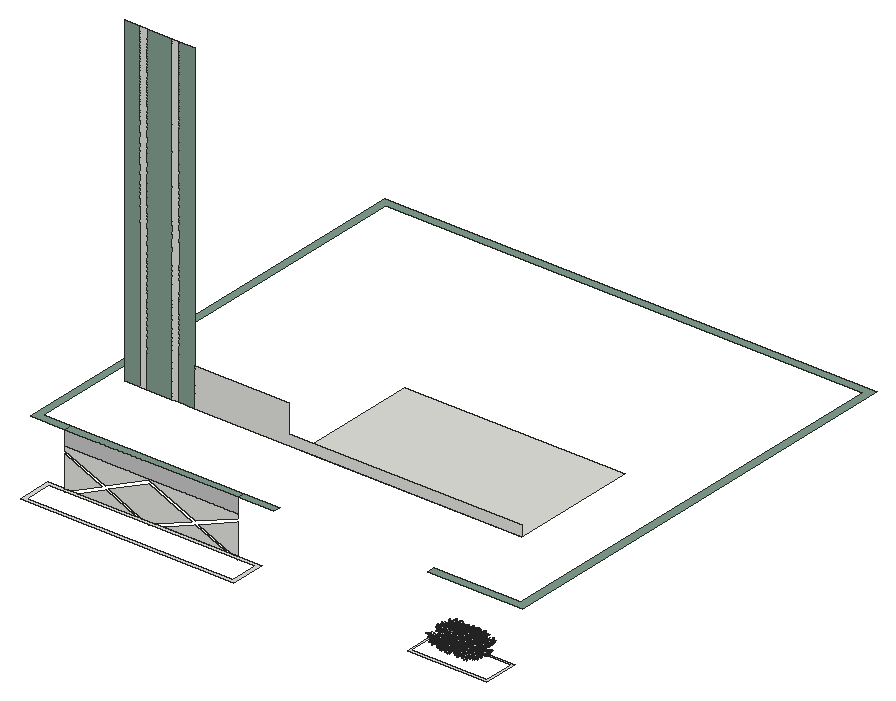
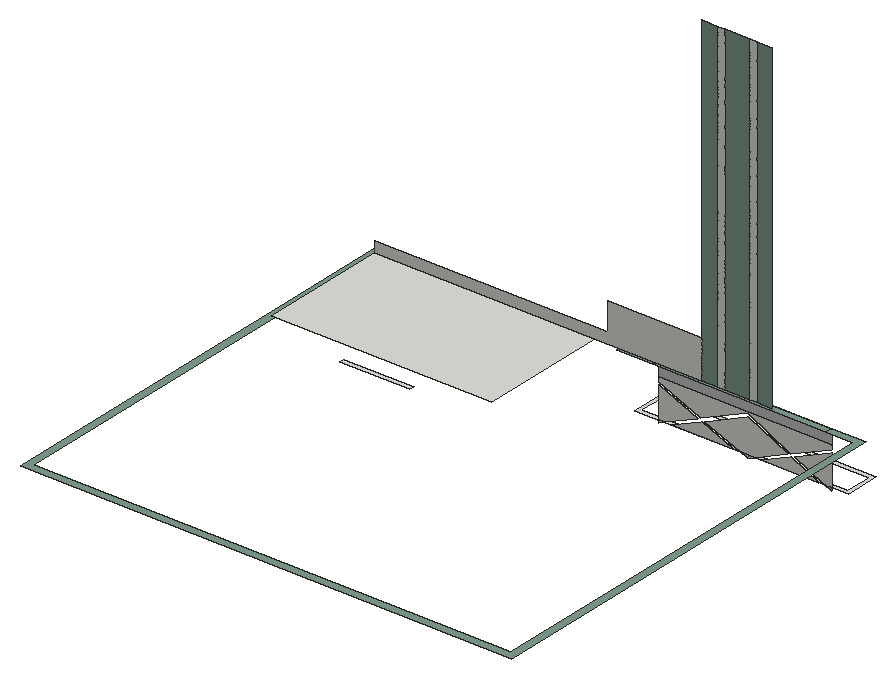
# SketchUp Ruby script. Lengths in inches.
U = 1.inch
M = Sketchup.active_model
def pt(a) = Geom::Point3d.new(a.map { |v| v * U })
def face(e, loops, mat)
  f = e.add_face(loops[0].map { |a| pt(a) })
  loops[1..].each { |l| e.add_face(l.map { |a| pt(a) }).erase! }
  f.material = f.back_material = mat if mat
  f
end
# faces: each face lists its corners as indices into pts; further lists are holes
def faces(e, pts, list, mat = nil) = list.each { |f| face(e, (f[0].is_a?(Array) ? f : [f]).map { |l| l.map { |i| pts[i] } }, mat) }
# xy, xz, yz: faces in a plane at the given z, y or x. An outline is a flat list of corners, or four numbers for a rectangle; further outlines are holes
def ring(l) = l.size == 4 ? [[l[0], l[1]], [l[2], l[1]], [l[2], l[3]], [l[0], l[3]]] : l.each_slice(2).to_a
def flat(e, list, mat, &to3) = list.each { |f| face(e, (f[0].is_a?(Array) ? f : [f]).map { |l| ring(l).map { |u, v| to3.(u, v) } }, mat) }
def xy(e, z, list, mat = nil) = flat(e, list, mat) { |x, y| [x, y, z] }
def xz(e, y, list, mat = nil) = flat(e, list, mat) { |x, z| [x, y, z] }
def yz(e, x, list, mat = nil) = flat(e, list, mat) { |y, z| [x, y, z] }
def lines(e, pts, list) = list.each { |a, b| e.add_line(pt(pts[a]), pt(pts[b])) }
# prism: a flat outline (further loops are holes) pulled along v
def prism(e, loops, v, mat = nil)
  f = face(e, loops, mat); d = Geom::Vector3d.new(v.map { |x| x * U })
  f.pushpull(f.normal.samedirection?(d) ? d.length : -d.length)
end
def box(e, o, s, mat = nil) = prism(e, [[o, [o[0] + s[0], o[1], o[2]], [o[0] + s[0], o[1] + s[1], o[2]], [o[0], o[1] + s[1], o[2]]]], [0, 0, s[2]], mat)
def at(x, y, z, deg = 0) = Geom::Transformation.translation(pt([x, y, z])) * Geom::Transformation.rotation(ORIGIN, Z_AXIS, deg.degrees)
def axes(o, x, y, z) = Geom::Transformation.new([*x, 0, *y, 0, *z, 0, *pt(o).to_a, 1])
def part(name) = M.definitions.add(name)
# library, detail: a bought-in or finely detailed component or shape, given as its bounding box
def library(name, o, s) = part(name).tap { |d| box(d.entities, o, s) }
def detail(e, o, s) = box(e.add_group.entities, o, s)
def put(e, d, t, mat = nil) = e.add_instance(d, t).tap { |i| i.material = mat if mat }
def group(e, t, mat = nil) = e.add_group.tap { |g| g.transformation = t; g.material = mat if mat }.entities
root = M.entities
M.materials.add("[Color H08]").color = [130, 158, 143]
M.materials.add("[Color M02]").color = [198, 198, 198]
c1 = part("Plane.003")
p = [[-13.75,10.1875,13.53],[-8.85,45.75,19.16],[-0.05,76.91,20.56],[0.09,-0.03,-0.02],[7.48,49.37,17.16],[14.16,9.16,9.9]]
faces(c1.entities,p,[[0,1,2,3],[4,5,3,2]])
c2 = part("spirea_leaf")
put(c2.entities,c1,at(0,0,0))
c3 = part("Plane.002")
p = [[-2.92,82.99,124.67],[-2.92,-0.79,0],[2.92,-0.79,0],[2.92,82.99,124.67],[2.92,149.28,292.15],[-2.92,149.28,292.15],
  [2.92,182.43,464.87],[-2.92,182.43,464.87]]
faces(c3.entities,p,[[0,1,2,3],[3,4,5,0],[5,4,6],[5,6,7]])
c4 = part("spirea_stem")
put(c4.entities,c3,at(0,0,0))
c5 = part("spirea_single")
put(c5.entities,c2,axes([61.07,82.24,152.17],[-0.04534,0.68195,-0.35141],[-0.74248,-0.12758,-0.15177],[-0.19302,0.33055,0.66639]))
put(c5.entities,c2,axes([59.72,73.38,127.91],[0.28617,0.56014,-0.10586],[-0.56688,0.26713,-0.11894],[-0.06012,0.14744,0.61766]))
put(c5.entities,c4,axes([60.19,1.84,0],[0.3441,0,0],[0,0.62,0],[0,0,0.62]))
put(c5.entities,c2,axes([59.67,34.88,53.33],[0.45126,0.21625,-0.53161],[-0.52806,0.42133,-0.27684],[0.2248,0.55563,0.41684]))
put(c5.entities,c2,axes([59.72,42.6,61.76],[0.43966,-0.56732,0.27467],[0.6265,0.43009,-0.11449],[-0.0692,0.28942,0.70855]))
put(c5.entities,c2,axes([60.64,103.19,225.26],[-0.35027,-0.4893,-0.00056],[0.48916,-0.35019,0.01365],[-0.01142,0.00749,0.60159]))
put(c5.entities,c2,axes([59.49,100.02,211.41],[0.59184,-0.32302,0],[0.323,0.59181,-0.00668],[0.0032,0.00586,0.67422]))
put(c5.entities,c2,axes([60.71,98.4,200.52],[0.37279,0.59177,-0.19096],[-0.61923,0.37358,-0.05117],[0.05663,0.18942,0.69752]))
put(c5.entities,c2,axes([60.46,79.17,144.19],[-0.69777,0.02304,-0.21354],[-0.09001,-0.69041,0.21963],[-0.195,0.23624,0.6627]))
put(c5.entities,c2,axes([59.53,75.43,133.01],[0.51977,-0.50179,-0.10513],[0.47164,0.52669,-0.18209],[0.201,0.06172,0.69914]))
put(c5.entities,c2,axes([61.85,65.23,103.75],[-0.33765,-0.67856,0.12705],[0.68306,-0.34887,-0.04799],[0.10005,0.09184,0.75641]))
put(c5.entities,c2,axes([59.93,92.9,176.87],[0.03118,-0.56709,0.29033],[0.62588,0.08155,0.09208],[-0.11899,0.28038,0.56044]))
put(c5.entities,c2,axes([60.8125,96.09,190.88],[-0.43546,0.45576,-0.27755],[-0.47188,-0.49616,-0.07437],[-0.24915,0.14314,0.62595]))
put(c5.entities,c2,axes([61.06,86.21,159.17],[0.68151,0.1886,0.10384],[-0.14294,0.65414,-0.24995],[-0.161,0.21757,0.66147]))
put(c5.entities,c2,axes([61.02,103.72,233.5],[0.15025,0.6695,-0.05975],[-0.66771,0.14162,-0.09212],[-0.07726,0.07802,0.67994]))
put(c5.entities,c2,axes([59.84,60.39,94.71],[0.69689,-0.19053,-0.10513],[0.16077,0.68848,-0.18209],[0.14666,0.15067,0.69914]))
put(c5.entities,c2,axes([60.35,111.25,265.8],[-0.44527,0.00464,-0.00041],[-0.00465,-0.44516,0.0101],[-0.00031,0.0101,0.44518]))
put(c5.entities,c2,axes([62.04,106.17,241.79],[0.58725,0,0],[0,0.58493,-0.0522],[0,0.0522,0.58493]))
put(c5.entities,c2,axes([61.05,108.11,252.87],[-0.04027,-0.58443,0.33381],[0.6723,-0.01918,0.04751],[-0.03168,0.33568,0.58389]))
c6 = part("spirea_noflower")
put(c6.entities,c4,axes([7.4375,15.95,0.02],[-0.05138,-0.02266,0],[0.04001,-0.09072,0.02017],[-0.00814,0.01846,0.09915]))
put(c6.entities,c2,axes([10.92,7.8,33.61],[0.09808,-0.04627,-0.02956],[0.03942,0.10146,-0.02804],[0.03822,0.0141,0.10476]))
put(c6.entities,c2,axes([10.66,8.28,28.22],[-0.09096,-0.06939,0.02274],[0.06684,-0.09374,-0.01869],[0.0294,-0.00154,0.11286]))
put(c6.entities,c2,axes([10.82,7.9375,40.67],[0.02156,-0.10964,0.01223],[0.11005,0.02051,-0.01012],[0.00764,0.01391,0.11128]))
put(c6.entities,c2,axes([10.02,10.22,17.07],[-0.11498,-0.02115,-0.02301],[0.02282,-0.11675,-0.00672],[-0.02136,-0.01089,0.11671]))
put(c6.entities,c2,axes([10.95,7.79,39.34],[0.02073,0.09465,-0.01601],[-0.09582,0.01943,-0.00921],[-0.00571,0.01757,0.09645]))
put(c6.entities,c2,axes([9.92,9.65,18.67],[0.00496,0.12531,-0.00176],[-0.12388,0.00463,-0.01903],[-0.01894,0.00249,0.12396]))
put(c6.entities,c2,axes([11.03,7.9,31.26],[-0.04507,0.08957,0.02798],[-0.0894,-0.05041,0.01738],[0.0285,-0.01651,0.09875]))
put(c6.entities,c2,axes([8.95,12.73,9.62],[-0.04645,-0.07719,-0.07798],[0.10968,-0.03512,-0.03057],[-0.00318,-0.0837,0.08474]))
put(c6.entities,c2,axes([10.44,9.32,22.8],[-0.00519,-0.10396,0.0013],[0.10345,-0.00529,-0.01033],[0.01038,0.00077,0.10358]))
put(c6.entities,c2,axes([9.33,11.85,11.22],[-0.10587,0.06223,0.02547],[-0.06429,-0.1076,-0.00432],[0.01971,-0.0167,0.12273]))
put(c6.entities,c2,axes([10.09,9.85,19.95],[0.08489,-0.07402,0.03033],[0.07003,0.09014,0.02399],[-0.03866,0.00075,0.11004]))
put(c6.entities,c2,axes([10.96,7.75,35.23],[-0.01497,-0.11683,-0.01129],[0.11725,-0.0154,0.00397],[-0.00539,-0.01068,0.11771]))
put(c6.entities,c2,axes([11.1,7.92,37.02],[-0.10922,0.00829,-0.01051],[-0.00995,-0.10807,0.01819],[-0.00895,0.019,0.10801]))
put(c6.entities,c2,axes([10.5,8.65,26.97],[0.0554,-0.10726,-0.03401],[0.10463,0.06305,-0.02842],[0.0414,-0.01582,0.11733]))
put(c6.entities,c2,axes([10.49,8.91,25.59],[0.10848,0.03623,-0.0334],[-0.034,0.11349,0.01266],[0.03566,-0.002,0.11367]))
put(c6.entities,c2,axes([10.54,9.18,23.68],[-0.10862,0.03606,-0.03314],[-0.03404,-0.11355,-0.01198],[-0.03521,-0.00146,0.11382]))
put(c6.entities,c2,axes([10.72,7.76,42.08],[-0.08769,-0.03868,0],[0.03843,-0.08714,0.01068],[-0.00431,0.00977,0.09524]))
put(c6.entities,c2,axes([10.85,7.87,43.91],[-0.03609,0.09811,0.03437],[-0.10225,-0.04006,0.00697],[0.01873,-0.02965,0.1043]))
put(c6.entities,c2,axes([10.98,7.84,46.08],[0.06679,0.02863,0.00008],[-0.02817,0.06574,-0.01287],[-0.00515,0.01179,0.07152]))
put(c6.entities,c2,axes([10.8,7.97,48.125],[-0.06893,0.0419,0.00009],[-0.04141,-0.06814,0.0122],[0.00642,0.01038,0.07974]))
put(c6.entities,c2,axes([10.94,7.82,49.1],[0.01894,-0.07016,0.00008],[0.05795,0.01569,0.04095],[-0.03956,-0.0106,0.06003]))
c7 = part("Spirea")
put(c7.entities,c5,axes([20.99,29.53,3.1875],[0.01954,-0.091,-0.02329],[0.08848,0.02778,-0.02423],[0.03497,-0.01946,0.07433]))
put(c7.entities,c5,axes([16.1875,23.97,1.65],[0.09656,0,0],[0,0.09656,0],[0,0,0.08111]))
put(c7.entities,c6,axes([35.43,25.1,-1.16],[-0.42763,0.26514,-0.05489],[-0.21558,-0.25326,0.32187],[0.16762,0.35071,0.27393]))
put(c7.entities,c6,axes([22.85,19.9,0.53],[0.4898,0.21094,-0.05818],[-0.15904,0.4504,0.20754],[0.15492,-0.20455,0.39699]))
put(c7.entities,c6,axes([25.64,17.62,5.32],[0.39778,0.28453,-0.05716],[-0.26298,0.39808,0.10688],[0.12818,-0.06625,0.39667]))
put(c7.entities,c6,axes([31.05,18.22,-1.16],[0.07698,0.49724,-0.05489],[-0.31736,0.09949,0.32187],[0.38833,-0.01726,0.27393]))
put(c7.entities,c5,axes([20.99,26.3,1.41],[0.06978,-0.07324,-0.00678],[0.06848,0.06856,-0.02532],[0.02721,0.01528,0.08112]))
put(c7.entities,c5,axes([22.49,26.46,1.43],[0.0904,0.01,-0.0061],[-0.01173,0.08633,-0.02277],[0.0039,0.02779,0.07293]))
put(c7.entities,c6,axes([30.45,32.2,-0.81],[0.02285,-0.56892,-0.06212],[0.15135,-0.06541,0.46198],[-0.55338,-0.04138,0.12379]))
put(c7.entities,c6,axes([21.91,22.81,-0.85],[-0.02216,0.50268,-0.05489],[-0.17773,0.05355,0.39666],[0.47473,0.04352,0.14594]))
put(c7.entities,c5,axes([30.1,30.77,0.36],[-0.1011,-0.04459,0],[0.04369,-0.09907,0.0185],[-0.00889,0.02016,0.09095]))
put(c7.entities,c5,axes([21.74,22.85,1.41],[0.07373,0.06926,-0.00678],[-0.06808,0.06896,-0.02532],[-0.01509,0.02732,0.08112]))
put(c7.entities,c5,axes([16.43,23,1.65],[0.06407,0.07017,0],[-0.07017,0.06407,0],[0,0,0.07982]))
put(c7.entities,c5,axes([17.07,18.375,1.34],[0.03932,0.08211,-0.00611],[-0.07957,0.0357,-0.02279],[-0.02155,0.01801,0.073]))
put(c7.entities,c5,axes([28.5,22.43,1.65],[-0.08829,0.05201,0],[-0.05201,-0.08829,0],[0,0,0.08608]))
put(c7.entities,c6,axes([28.93,29.38,-2.32],[-0.56896,-0.02186,-0.06212],[-0.04199,-0.37401,0.36423],[-0.06468,0.43508,0.30998]))
put(c7.entities,c5,axes([30.22,28.68,0.43],[-0.09325,-0.03922,-0.00678],[0.04003,-0.09171,-0.01417],[-0.00078,-0.01869,0.08379]))
put(c7.entities,c5,axes([22.83,20.65,3.32],[-0.01797,0.0853,0],[-0.08403,-0.01771,-0.01259],[-0.01466,-0.00309,0.07213]))
put(c7.entities,c6,axes([24.5,33.17,-1.16],[-0.36679,-0.34444,-0.05489],[0.18883,-0.27379,0.32187],[-0.29538,0.25268,0.27393]))
put(c7.entities,c6,axes([16.17,23.58,-0.85],[0.44167,0.24105,-0.05489],[-0.0301,0.18317,0.39666],[0.24793,-0.40717,0.14594]))
put(c7.entities,c6,axes([15.32,23.08,-1.16],[0.43965,-0.24471,-0.05489],[0.20342,0.26314,0.32187],[-0.15091,-0.35822,0.27393]))
put(c7.entities,c6,axes([25.22,18.48,-2.32],[0.43489,0.36751,-0.06212],[-0.19718,0.32058,0.36423],[0.31883,-0.30303,0.30998]))
put(c7.entities,c6,axes([17.47,17.85,-1.16],[0.50022,0.05434,-0.05489],[0.01396,0.3323,0.32187],[0.08384,-0.37956,0.27393]))
put(c7.entities,c6,axes([19.68,35.94,-1.16],[-0.12258,-0.488,-0.05489],[0.30682,-0.12838,0.32187],[-0.38507,0.05305,0.27393]))
put(c7.entities,c5,axes([20.21,32.32,1.65],[0.059,-0.08211,0],[0.08211,0.059,0],[0,0,0.08493]))
put(c7.entities,c5,axes([30.73,22.42,1.41],[-0.10081,0.00845,-0.00678],[-0.00569,-0.09674,-0.02532],[-0.01021,-0.02949,0.08112]))
put(c7.entities,c6,axes([19.68,37.38,0.39],[-0.15639,-0.58365,0],[0.58365,-0.15639,0],[0,0,0.50756]))
put(c7.entities,c6,axes([14.16,35.57,1.53],[-0.16219,-0.57166,-0.08263],[0.57944,-0.1644,0],[-0.02685,-0.09464,0.49914]))
put(c7.entities,c6,axes([17.58,28.45,-2.32],[0.19381,-0.53538,-0.06212],[0.36907,0.07371,0.36423],[-0.39482,-0.1939,0.30998]))
xy(root,16.375,[[[21.01,42.875,281.76,85.1875],[25.26,47.13,277.5,80.93]],[[493.5625,43.3125,590.375,85.1875],[495.57,45.32,588.37,83.18]]])
xy(root,81,[[0,85.1875,42.01,85.1875,42.01,94.1875,9,94.1875,9,616.1875,591,616.1875,591,94.1875,484.36,94.1875,484.36,85.1875,600,85.1875,600,625.1875,0,625.1875],[42.01,85.1875,253.1,94.1875],[253.1,85.1875,296.4375,94.1875]],"[Color H08]")
xy(root,101.5625,[[380.7,299.125,465.83,305.125]])
xy(root,118.4375,[[285.75,142.1875,554.1875,299.125]])
xz(root,85.1875,[[42.01,12.82,42.01,16.375,49.44,16.375],[253.1,12.82,245.17,16.375,253.1,16.375],[143.93,12.83,135.91,16.375,144.11,16.375,144.11,12.91],[144.11,12.91,144.11,16.375,152.53,16.375],[42.01,16.375,49.44,16.375,86.99,34.34,42.01,54.29],
  [57.43,16.375,127.49,16.375,91.13,32.5],[135.91,16.375,152.53,16.375,196.33,34.44,144.11,57.85,95.125,34.41],[161.86,16.375,236.65,16.375,200.67,32.5],[245.17,16.375,253.1,16.375,253.1,54.29,205.09,34.34],[90.97,36.24,144.11,61.67,200.77,36.27,253.1,57.86,253.1,63.13,42.01,63.13,42.01,57.9]])
xz(root,85.1875,[[42.01,63.13,253.1,81]],"[Color M02]")
xz(root,142.1875,[[87.99,118.4375,96.21,512.9375],[126.87,118.4375,135.08,512.9375],[155.14,118.4375,554.1875,118.4375,554.1875,131.51,269.375,131.51,269.375,165.45,155.14,165.45]])
xz(root,142.1875,[[69,118.4375,87.99,512.9375],[96.21,118.4375,126.87,512.9375],[135.08,118.4375,155.14,512.9375]],"[Color H08]")
put(root,c7,at(500.92,47.88,15.71))
put(root,c7,at(521.79,47.88,15.71))
